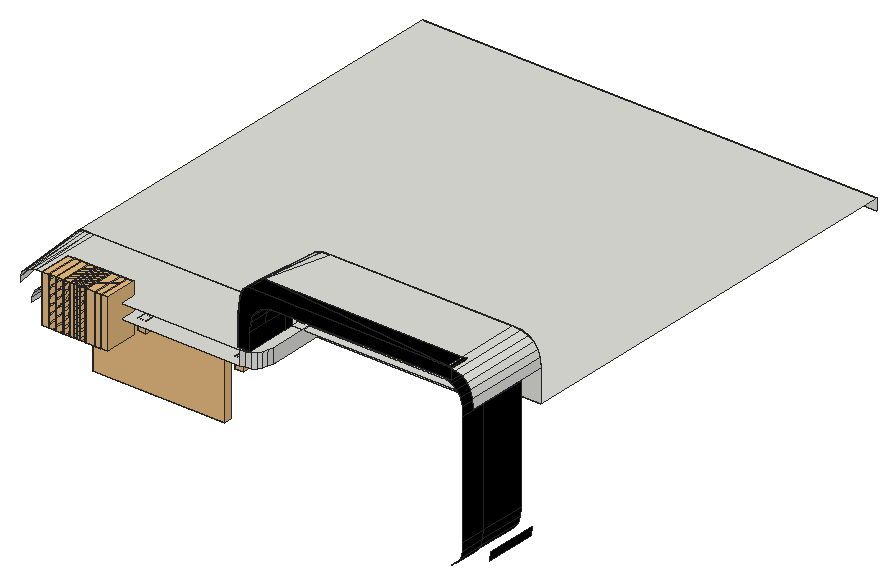
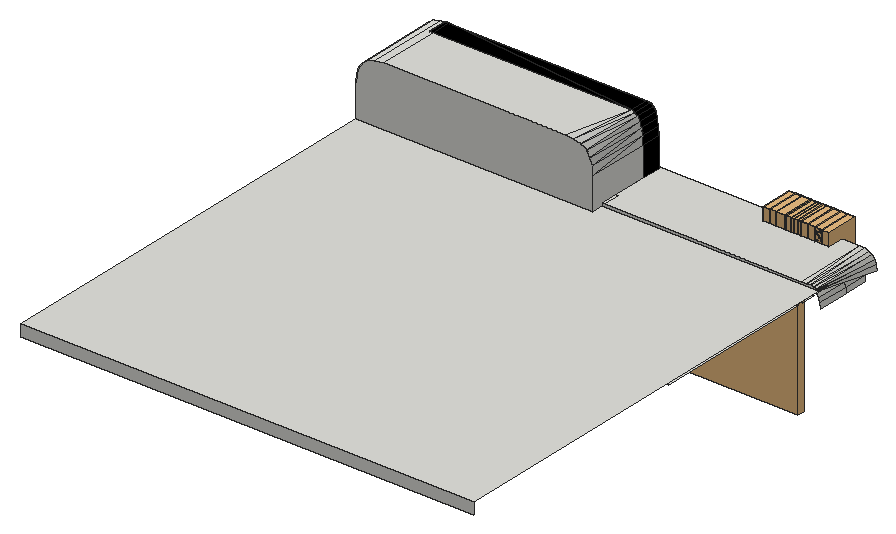
# SketchUp Ruby script. Lengths in inches.
U = 1.inch
M = Sketchup.active_model
def pt(a) = Geom::Point3d.new(a.map { |v| v * U })
def face(e, loops, mat)
  f = e.add_face(loops[0].map { |a| pt(a) })
  loops[1..].each { |l| e.add_face(l.map { |a| pt(a) }).erase! }
  f.material = f.back_material = mat if mat
  f
end
# faces: each face lists its corners as indices into pts; further lists are holes
def faces(e, pts, list, mat = nil) = list.each { |f| face(e, (f[0].is_a?(Array) ? f : [f]).map { |l| l.map { |i| pts[i] } }, mat) }
# xy, xz, yz: faces in a plane at the given z, y or x. An outline is a flat list of corners, or four numbers for a rectangle; further outlines are holes
def ring(l) = l.size == 4 ? [[l[0], l[1]], [l[2], l[1]], [l[2], l[3]], [l[0], l[3]]] : l.each_slice(2).to_a
def flat(e, list, mat, &to3) = list.each { |f| face(e, (f[0].is_a?(Array) ? f : [f]).map { |l| ring(l).map { |u, v| to3.(u, v) } }, mat) }
def xy(e, z, list, mat = nil) = flat(e, list, mat) { |x, y| [x, y, z] }
def xz(e, y, list, mat = nil) = flat(e, list, mat) { |x, z| [x, y, z] }
def yz(e, x, list, mat = nil) = flat(e, list, mat) { |y, z| [x, y, z] }
def lines(e, pts, list) = list.each { |a, b| e.add_line(pt(pts[a]), pt(pts[b])) }
# prism: a flat outline (further loops are holes) pulled along v
def prism(e, loops, v, mat = nil)
  f = face(e, loops, mat); d = Geom::Vector3d.new(v.map { |x| x * U })
  f.pushpull(f.normal.samedirection?(d) ? d.length : -d.length)
end
def box(e, o, s, mat = nil) = prism(e, [[o, [o[0] + s[0], o[1], o[2]], [o[0] + s[0], o[1] + s[1], o[2]], [o[0], o[1] + s[1], o[2]]]], [0, 0, s[2]], mat)
def at(x, y, z, deg = 0) = Geom::Transformation.translation(pt([x, y, z])) * Geom::Transformation.rotation(ORIGIN, Z_AXIS, deg.degrees)
def axes(o, x, y, z) = Geom::Transformation.new([*x, 0, *y, 0, *z, 0, *pt(o).to_a, 1])
def part(name) = M.definitions.add(name)
# library, detail: a bought-in or finely detailed component or shape, given as its bounding box
def library(name, o, s) = part(name).tap { |d| box(d.entities, o, s) }
def detail(e, o, s) = box(e.add_group.entities, o, s)
def put(e, d, t, mat = nil) = e.add_instance(d, t).tap { |i| i.material = mat if mat }
def group(e, t, mat = nil) = e.add_group.tap { |g| g.transformation = t; g.material = mat if mat }.entities
root = M.entities
M.materials.add("[Color M09]").color = [0, 0, 0]
c1 = library("Curtains",[0,0,0],[121.73,8.19,117.22])
c2 = library("Hanging Plant",[-3.24,-2.02,-0.87],[34.15,22.68,50.98])
c3 = library("IES Light",[-4.45,-4.45,-12],[8.9,8.9,12])
xy(root,272.125,[[796.3125,260.875,796.3125,453.4375,996.66,453.4375,996.66,266.1,978.47,266.1,978.47,260.875]])
xy(root,279,[[806.73,202.125,806.73,226.5,1009.83,226.5,1011.01,227.13,1012.14,227.86,1013.21,228.68,1014.21,229.58,1015.125,230.5625,1015.96,231.61,1016.71,232.73,1017.36,233.91,1017.92,235.13,1018.375,236.39,1018.73,237.69,1018.97,239.01,1018.97,278.875,1029.53,278.875,1029.53,221.83,1028.98,215.81,1027.34,210.88,1024.61,207.05,1020.77,204.3125,1015.85,202.67,1009.83,202.125],[806.73,227.5,806.73,260.875,1003.53,260.875,1003.53,278.875,1017.97,278.875,1017.97,239.01,1017.7,237.83,1017.35,236.67,1016.91,235.54,1016.4,234.44,1015.8125,233.39,1015.15,232.375,1014.41,231.41,1013.61,230.5,1012.75,229.65,1011.83,228.87,1010.85,228.15,1009.83,227.5],[1029.53,278.875,1197.4375,527.4375]])
xy(root,291,[[777.4375,278.875,1006.27,278.875,1006.27,290.7,1257.4375,290.7,1257.4375,734.875,777.4375,734.875]])
xy(root,294,[[794.73,202.125,1009.83,202.125,1015.85,202.67,1020.77,204.3125,1024.61,207.05,1027.34,210.88,1028.98,215.81,1029.53,221.83,1029.53,260.875,1018.27,260.875,1018.27,204.5,1006.27,204.5,1006.27,260.875,1003.53,260.875,1003.53,278.875,794.73,278.875],[1003.53,260.875,1006.27,278.875],[1018.27,260.875,1029.53,278.875],[1029.53,260.875,1194.29,268.8125],[1029.53,269.8125,1194.29,278.875]])
xy(root,306,[[1018.27,260.875,1204,278.875]])
xy(root,342,[[1047.51,204.5,1047.51,222.09,1216.2,206.05,1216.2,224.875,1232.38,224.875,1232.38,204.5],[1216.2,206.05,1047.51,222.09,1047.51,248.03,1216.2,231.99],[1216.2,232.99,1047.51,249.03,1047.51,278.875,1216.2,278.875]],"[Color M09]")
xy(root,354,[[1018.27,224.875,1228.2,224.875,1228.2,290.7,1035.51,290.7]])
xy(root,354,[[1018.27,204.5,1232.38,204.5,1232.38,204.91,1228.2,204.91,1018.27,224.875],[1228.2,204.91,1228.2,224.875,1018.27,224.875],[1228.2,204.91,1232.38,224.875]],"[Color M09]")
xz(root,204.5,[[1006.27,294,1018.27,294,1018.27,312.76,1019.09,321.69,1021.52,329,1025.58,334.69,1031.27,338.75,1038.58,341.1875,1047.51,342,1232.38,342,1232.38,354,1018.27,354,1014.61,353.1875,1011.61,350.75,1009.27,346.69,1007.61,341,1006.61,333.69,1006.27,324.76]],"[Color M09]")
xz(root,278.875,[[777.4375,291,777.92,291.92,779.36,292.67,781.76,293.25,785.125,293.67,789.45,293.92,794.73,294,1006.27,294,1006.27,291]])
xz(root,290.7,[[1006.27,291,1006.27,324.76,1007.09,333.69,1009.52,341,1013.58,346.69,1019.27,350.75,1026.58,353.1875,1035.51,354,1228.2,354,1237.13,353.1875,1244.44,350.75,1250.13,346.69,1254.1875,341,1256.625,333.69,1257.4375,324.76,1257.4375,291]])
xz(root,734.875,[[777.4375,279,1257.4375,291]])
yz(root,1006.27,[[278.875,291,278.875,294,224.875,294,224.875,324.76,290.7,324.76,290.7,291]])
yz(root,1006.27,[[204.5,294,224.875,324.76]],"[Color M09]")
yz(root,1018.27,[[204.5,294,250.8125,312.76],[251.8125,294,260.875,294,260.875,306,278.875,306,278.875,312.76,251.8125,312.76]],"[Color M09]")
yz(root,1029.53,[[221.83,279,278.875,294]])
yz(root,1232.38,[[204.5,342,224.875,354]],"[Color M09]")
yz(root,1245.4375,[[203.27,193.12,229.2,312.76],[230.2,193.12,278.875,312.76]],"[Color M09]")
p = [[1238.13,203.96,171.19],[1238.13,229.9,171.19],[1232.44,230.44,167.125],[1232.44,204.5,167.125],[1232.44,278.875,167.125],[1232.44,231.44,167.125],
  [1238.13,230.9,171.19],[1238.13,278.875,171.19],[1257.4375,224.875,179.24],[1256.625,224.875,170.31],[1256.625,278.875,170.31],[1257.4375,278.875,179.24],
  [1242.1875,203.58,176.87],[1242.1875,229.51,176.87],[1242.1875,230.51,176.87],[1242.1875,278.875,176.87],[1244.625,203.34,184.18],[1244.625,229.28,184.18],
  [1244.625,230.28,184.18],[1244.625,278.875,184.18],[1245.4375,203.27,193.12],[1245.4375,229.2,193.12],[1245.4375,230.2,193.12],[1245.4375,278.875,193.12],
  [789.4375,202.125,261.71],[789.4375,226.5,261.71],[789.92,226.5,266.99],[789.92,202.125,266.99],[789.92,260.875,266.99],[789.92,227.5,266.99],
  [789.4375,227.5,261.71],[789.4375,260.875,261.71],[791.36,226.5,271.3125],[791.36,202.125,271.3125],[791.36,260.875,271.3125],[791.36,227.5,271.3125],
  [793.76,226.5,274.68],[793.76,202.125,274.68],[793.76,260.875,274.68],[793.76,227.5,274.68],[797.125,226.5,277.08],[797.125,202.125,277.08],
  [797.125,260.875,277.08],[797.125,227.5,277.08],[777.4375,278.875,291],[777.4375,202.125,276.71],[777.92,202.125,281.99],[801.45,226.5,278.52],
  [801.45,202.125,278.52],[801.45,260.875,278.52],[801.45,227.5,278.52],[806.73,226.5,279],[806.73,202.125,279],[806.73,260.875,279],
  [806.73,227.5,279],[1209.02,260.875,283.48],[1209.02,268.8125,283.48],[1209.4375,268.8125,278.86],[1209.4375,260.875,278.86],[1209.4375,278.875,278.86],
  [1209.4375,269.8125,278.86],[1209.02,269.8125,283.48],[1209.02,278.875,283.48],[1015.85,202.67,279],[1015.85,202.67,294],[1009.83,202.125,294],
  [1009.83,202.125,279],[1020.77,204.3125,279],[1020.77,204.3125,294],[1024.61,207.05,279],[1024.61,207.05,294],[1027.34,210.88,279],
  [1027.34,210.88,294],[1028.98,215.81,279],[1028.98,215.81,294],[1029.53,221.83,279],[1029.53,221.83,294],[777.92,278.875,291.92],
  [779.36,202.125,286.3125],[1207.75,260.875,287.27],[1207.75,268.8125,287.27],[1207.75,269.8125,287.27],[1207.75,278.875,287.27],[779.36,278.875,292.67],
  [781.76,202.125,289.68],[1205.65,260.875,290.21],[1205.65,268.8125,290.21],[1205.65,269.8125,290.21],[1205.65,278.875,290.21],[1220.95,278.875,293.89],
  [1220.95,260.875,293.89],[1221.4375,260.875,288.5625],[1221.4375,278.875,288.5625],[781.76,278.875,293.25],[785.125,202.125,292.08],[1202.71,260.875,292.32],
  [1202.71,268.8125,292.32],[1202.71,269.8125,292.32],[1202.71,278.875,292.32],[785.125,278.875,293.67],[789.45,202.125,293.52],[1198.92,260.875,293.58],
  [1198.92,268.8125,293.58],[1198.92,269.8125,293.58],[1198.92,278.875,293.58],[789.45,278.875,293.92],[794.73,202.125,294],[1194.29,260.875,294],
  [1194.29,268.8125,294],[1194.29,269.8125,294],[1194.29,278.875,294],[794.73,278.875,294],[1219.5,278.875,298.25],[1219.5,260.875,298.25],
  [1217.08,278.875,301.64],[1217.08,260.875,301.64],[1213.6875,278.875,304.0625],[1213.6875,260.875,304.0625],[1209.33,278.875,305.52],[1209.33,260.875,305.52],
  [1204,278.875,306],[1204,260.875,306],[1244.625,203.34,321.69],[1244.625,229.28,321.69],[1245.4375,229.2,312.76],[1245.4375,203.27,312.76],
  [1018.27,204.5,312.76],[1018.27,224.875,312.76],[1019.09,224.8,321.69],[1019.09,204.5,321.69],[1018.27,250.8125,312.76],[1019.09,250.74,321.69],
  [1245.4375,278.875,312.76],[1245.4375,230.2,312.76],[1244.625,230.28,321.69],[1244.625,278.875,321.69],[1019.09,278.875,321.69],[1019.09,251.74,321.69],
  [1018.27,251.8125,312.76],[1018.27,278.875,312.76],[1242.1875,203.58,329],[1242.1875,229.51,329],[1021.52,224.57,329],[1021.52,204.5,329],
  [1021.52,250.5,329],[1242.1875,230.51,329],[1242.1875,278.875,329],[1021.52,278.875,329],[1021.52,251.5,329],[1257.4375,202.125,324.76],
  [1257.4375,290.7,324.76],[1256.625,290.7,333.69],[1256.625,202.2,333.69],[1006.61,224.875,333.69],[1006.27,224.875,324.76],[1006.27,204.5,324.76],
  [1006.61,204.5,333.69],[1006.27,290.7,324.76],[1007.09,290.7,333.69],[1238.13,203.96,334.69],[1238.13,229.9,334.69],[1025.58,224.18,334.69],
  [1025.58,204.5,334.69],[1025.58,250.12,334.69],[1238.13,230.9,334.69],[1238.13,278.875,334.69],[1025.58,278.875,334.69],[1025.58,251.12,334.69],
  [1254.1875,290.7,341],[1254.1875,202.43,341],[1007.61,224.875,341],[1007.61,204.5,341],[1009.52,290.7,341],[1232.44,204.5,338.75],
  [1232.44,230.44,338.75],[1031.27,223.64,338.75],[1031.27,204.5,338.75],[1031.27,249.58,338.75],[1232.44,231.44,338.75],[1232.44,278.875,338.75],
  [1031.27,278.875,338.75],[1031.27,250.58,338.75],[1038.58,222.94,341.1875],[1038.58,204.5,341.1875],[1225.13,205.2,341.1875],[1225.13,231.14,341.1875],
  [1038.58,248.88,341.1875],[1225.13,232.14,341.1875],[1225.13,278.875,341.1875],[1038.58,278.875,341.1875],[1038.58,249.88,341.1875],[1250.13,290.7,346.69],
  [1250.13,202.82,346.69],[1009.27,224.875,346.69],[1009.27,204.5,346.69],[1013.58,290.7,346.69],[1047.51,222.09,342],[1047.51,204.5,342],
  [1216.2,224.875,342],[1216.2,231.99,342],[1216.2,206.05,342],[1047.51,248.03,342],[1216.2,232.99,342],[1216.2,278.875,342],
  [1047.51,278.875,342],[1047.51,249.03,342],[1244.44,290.7,350.75],[1244.44,203.36,350.75],[1011.61,224.875,350.75],[1011.61,204.5,350.75],
  [1019.27,290.7,350.75],[1237.13,290.7,353.1875],[1237.13,204.06,353.1875],[1014.61,224.875,353.1875],[1014.61,204.5,353.1875],[1026.58,290.7,353.1875],
  [1228.2,290.7,354],[1228.2,224.875,354],[1228.2,204.91,354],[1018.27,224.875,354],[1018.27,204.5,354],[1035.51,290.7,354],
  [1026.22,302.8,279],[1026.22,278.875,279]]
faces(root,p,[[0,1,2,3],[4,5,6,7],[8,9,10,11],[12,13,1,0],[7,6,14,15],[16,17,13,12],[15,14,18,19],[20,21,17,16],
  [19,18,22,23],[122,123,124,125],[126,127,128,129],[128,127,130,131],[132,133,134,135],[136,137,138,139],[140,141,123,122],[129,128,142,143],
  [142,128,131,144],[135,134,145,146],[147,148,137,136],[153,154,155,156],[159,160,141,140],[143,142,161,162],[161,142,144,163],[146,145,164,165],
  [166,167,148,147],[170,153,156,171],[173,174,160,159],[162,161,175,176],[161,163,177,175],[165,164,178,179],[180,181,167,166],[176,175,182,183],
  [184,185,174,173],[182,175,177,186],[179,178,187,188],[189,190,181,180],[193,170,171,194],[183,182,196,197],[198,199,185,184,200],[196,182,186,201],
  [188,187,202,203],[204,205,190,189],[208,193,194,209],[213,208,209,214],[219,213,214,220]],"[Color M09]")
faces(root,p,[[24,25,26,27],[28,29,30,31],[27,26,32,33],[34,35,29,28],[33,32,36,37],[38,39,35,34],[37,36,40,41],[42,43,39,38],
  [44,45,46],[41,40,47,48],[49,50,43,42],[48,47,51,52],[53,54,50,49],[55,56,57,58],[59,60,61,62],[63,64,65,66],
  [67,68,64,63],[69,70,68,67],[71,72,70,69],[73,74,72,71],[75,76,74,73],[77,44,46],[77,46,78],[79,80,56,55],
  [62,61,81,82],[83,77,78],[83,78,84],[85,86,80,79],[82,81,87,88],[89,90,91,92],[93,83,84],[93,84,94],
  [95,96,86,85],[88,87,97,98],[99,93,94],[99,94,100],[101,102,96,95],[98,97,103,104],[105,99,100],[105,100,106],
  [107,108,102,101],[104,103,109,110],[111,105,106],[112,113,90,89],[114,115,113,112],[116,117,115,114],[118,119,117,116],[120,121,119,118],
  [149,150,151,152],[154,153,157],[153,158,157],[152,151,168,169],[153,170,158],[170,172,158],[169,168,191,192],[170,193,172],
  [193,195,172],[192,191,206,207],[193,208,195],[208,210,195],[207,206,211,212],[208,213,210],[213,215,210],[212,211,216,217,218],
  [213,219,215],[219,221,215]])
lines(root,p,[[222,223]])
put(root,c1,axes([796.76,273.6875,167.73],[1.15065,0,0],[0,1,0],[0,0,0.8928]))
put(root,c2,at(838.8,215.52,257.0625,-90))
put(root,c2,at(849.73,215.52,257.0625,-90))
put(root,c2,at(816.42,215.52,257.0625,-90))
put(root,c2,at(856.48,215.52,257.0625,-90))
put(root,c2,at(830.92,215.52,257.0625,-90))
put(root,c2,at(823.55,215.52,257.0625,-90))
put(root,c2,at(863.17,215.52,257.0625,-90))
put(root,c3,at(819.66,247.99,279))
put(root,c3,at(819.66,216.8,279))
put(root,c3,at(897.98,247.99,279))
put(root,c3,at(897.98,216.8,279))
put(root,c3,at(1001.05,247.99,279))
put(root,c3,at(1001.05,216.8,279))
put(root,c3,at(1060.59,255.24,342))
put(root,c3,at(1060.59,224.05,342))
put(root,c3,at(1117.78,255.24,342))
put(root,c3,at(1117.78,224.05,342))
put(root,c3,at(1174.97,255.24,342))
put(root,c3,at(1174.97,224.05,342))
put(root,c3,at(1232.15,255.24,342))
put(root,c3,at(1232.15,224.05,342))
